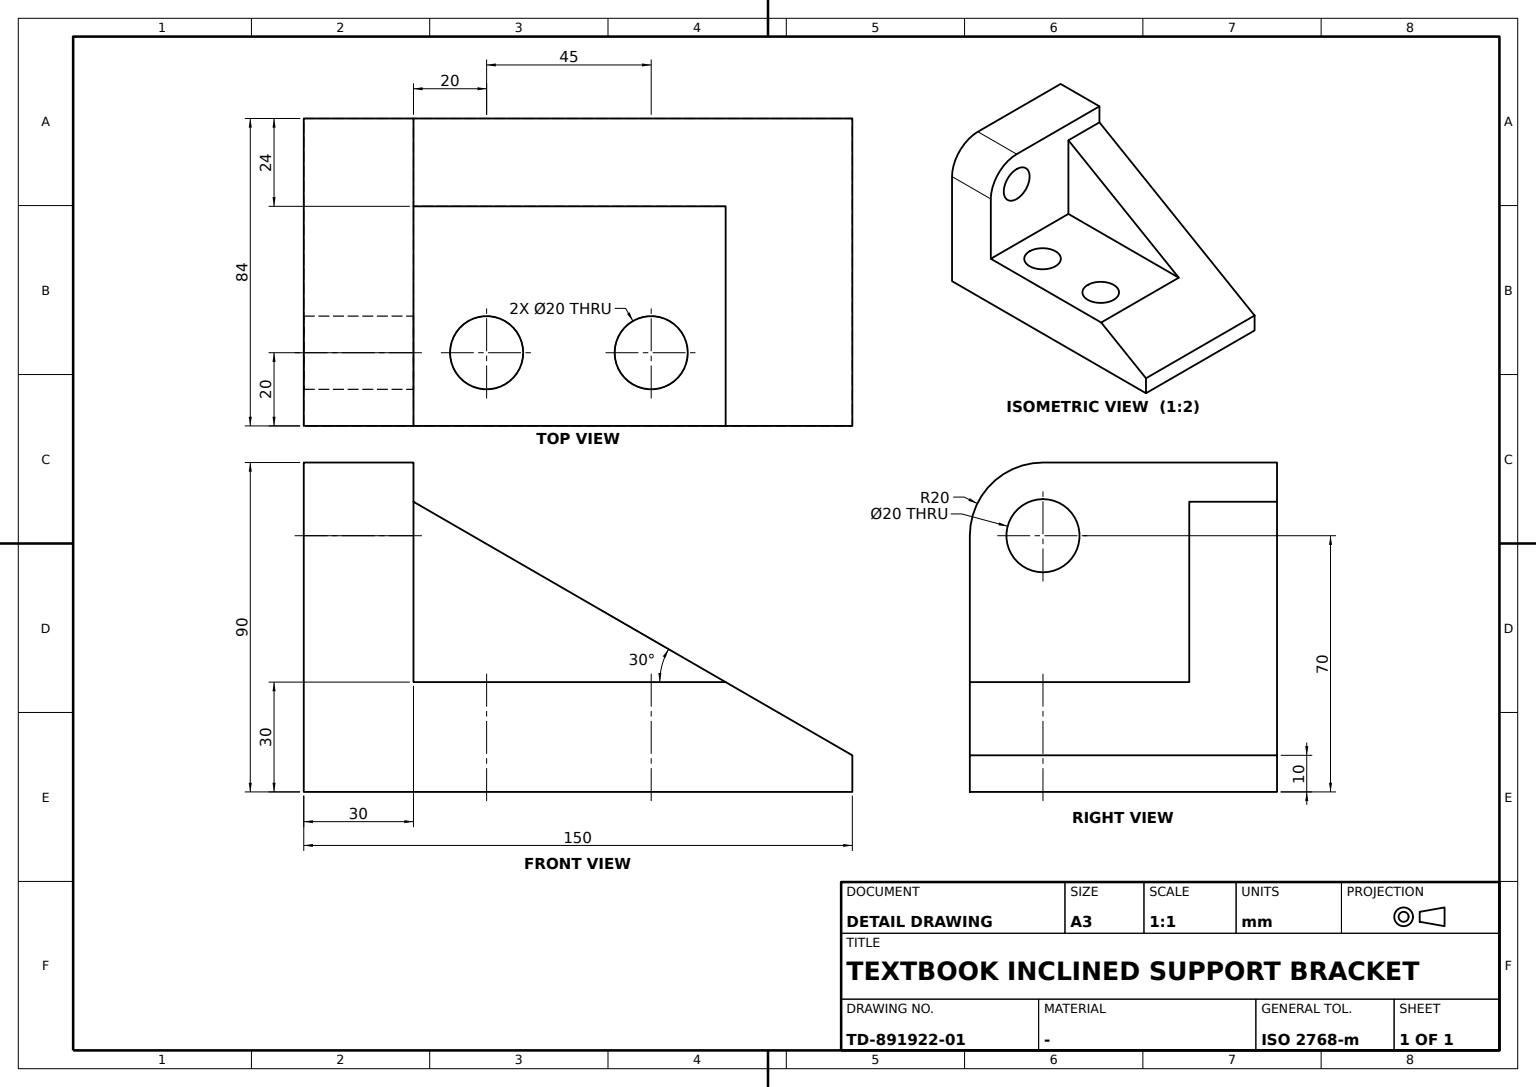
ISO-10303-21;
HEADER;
FILE_DESCRIPTION((''),'2;1');
FILE_NAME('','',(''),(''),'','','');
FILE_SCHEMA(('AUTOMOTIVE_DESIGN'));
ENDSEC;
DATA;
#1=APPLICATION_CONTEXT('');
#2=PRODUCT_CONTEXT('',#1,'mechanical');
#3=PRODUCT('','','',(#2));
#4=PRODUCT_DEFINITION_FORMATION('','',#3);
#5=PRODUCT_DEFINITION_CONTEXT('',#1,'design');
#6=PRODUCT_DEFINITION('','',#4,#5);
#7=PRODUCT_DEFINITION_SHAPE('','',#6);
#8=(LENGTH_UNIT()NAMED_UNIT(*)SI_UNIT(.MILLI.,.METRE.));
#9=(NAMED_UNIT(*)PLANE_ANGLE_UNIT()SI_UNIT($,.RADIAN.));
#10=(NAMED_UNIT(*)SI_UNIT($,.STERADIAN.)SOLID_ANGLE_UNIT());
#11=UNCERTAINTY_MEASURE_WITH_UNIT(LENGTH_MEASURE(0.005),#8,'distance_accuracy_value','');
#12=(GEOMETRIC_REPRESENTATION_CONTEXT(3)GLOBAL_UNCERTAINTY_ASSIGNED_CONTEXT((#11))GLOBAL_UNIT_ASSIGNED_CONTEXT((#8,#9,#10))REPRESENTATION_CONTEXT('',''));
#13=CARTESIAN_POINT('',(30.,-22.,60.));
#14=VERTEX_POINT('',#13);
#15=CARTESIAN_POINT('',(0.,-22.,60.));
#16=VERTEX_POINT('',#15);
#17=DIRECTION('',(1.,0.,0.));
#18=VECTOR('',#17,1000.);
#19=LINE('',#15,#18);
#20=EDGE_CURVE('',#14,#16,#19,.F.);
#21=ORIENTED_EDGE('',*,*,#20,.F.);
#22=CARTESIAN_POINT('',(30.,-22.,80.));
#23=VERTEX_POINT('',#22);
#24=CARTESIAN_POINT('',(30.,-22.,70.));
#25=DIRECTION('',(0.,1.,0.));
#26=AXIS2_PLACEMENT_3D('',#24,#17,#25);
#27=CIRCLE('',#26,10.);
#28=EDGE_CURVE('',#14,#23,#27,.T.);
#29=ORIENTED_EDGE('',*,*,#28,.T.);
#30=CARTESIAN_POINT('',(0.,-22.,80.));
#31=VERTEX_POINT('',#30);
#32=LINE('',#30,#18);
#33=EDGE_CURVE('',#31,#23,#32,.T.);
#34=ORIENTED_EDGE('',*,*,#33,.F.);
#35=CARTESIAN_POINT('',(0.,-22.,70.));
#36=AXIS2_PLACEMENT_3D('',#35,#17,#25);
#37=CIRCLE('',#36,10.);
#38=EDGE_CURVE('',#16,#31,#37,.T.);
#39=ORIENTED_EDGE('',*,*,#38,.F.);
#40=EDGE_LOOP('',(#21,#29,#34,#39));
#41=FACE_BOUND('',#40,.T.);
#42=DIRECTION('',(0.,0.,-1.));
#43=AXIS2_PLACEMENT_3D('',#35,#17,#42);
#44=CYLINDRICAL_SURFACE('',#43,10.);
#45=ADVANCED_FACE('',(#41),#44,.F.);
#46=CARTESIAN_POINT('',(85.,-22.,0.));
#47=VERTEX_POINT('',#46);
#48=CARTESIAN_POINT('',(105.,-22.,0.));
#49=VERTEX_POINT('',#48);
#50=CARTESIAN_POINT('',(95.,-22.,0.));
#51=DIRECTION('',(0.,0.,1.));
#52=AXIS2_PLACEMENT_3D('',#50,#51,#17);
#53=CIRCLE('',#52,10.);
#54=EDGE_CURVE('',#47,#49,#53,.T.);
#55=ORIENTED_EDGE('',*,*,#54,.T.);
#56=EDGE_CURVE('',#49,#47,#53,.T.);
#57=ORIENTED_EDGE('',*,*,#56,.T.);
#58=EDGE_LOOP('',(#55,#57));
#59=FACE_BOUND('',#58,.T.);
#60=CARTESIAN_POINT('',(0.,-42.,0.));
#61=VERTEX_POINT('',#60);
#62=CARTESIAN_POINT('',(0.,42.,0.));
#63=VERTEX_POINT('',#62);
#64=VECTOR('',#25,1000.);
#65=LINE('',#60,#64);
#66=EDGE_CURVE('',#61,#63,#65,.T.);
#67=ORIENTED_EDGE('',*,*,#66,.T.);
#68=CARTESIAN_POINT('',(150.,42.,0.));
#69=VERTEX_POINT('',#68);
#70=LINE('',#62,#18);
#71=EDGE_CURVE('',#63,#69,#70,.T.);
#72=ORIENTED_EDGE('',*,*,#71,.T.);
#73=CARTESIAN_POINT('',(150.,-42.,0.));
#74=VERTEX_POINT('',#73);
#75=LINE('',#73,#64);
#76=EDGE_CURVE('',#74,#69,#75,.T.);
#77=ORIENTED_EDGE('',*,*,#76,.F.);
#78=LINE('',#60,#18);
#79=EDGE_CURVE('',#61,#74,#78,.T.);
#80=ORIENTED_EDGE('',*,*,#79,.F.);
#81=EDGE_LOOP('',(#67,#72,#77,#80));
#82=FACE_BOUND('',#81,.T.);
#83=CARTESIAN_POINT('',(60.,-22.,0.));
#84=VERTEX_POINT('',#83);
#85=CARTESIAN_POINT('',(40.,-22.,0.));
#86=VERTEX_POINT('',#85);
#87=CARTESIAN_POINT('',(50.,-22.,0.));
#88=AXIS2_PLACEMENT_3D('',#87,#51,#17);
#89=CIRCLE('',#88,10.);
#90=EDGE_CURVE('',#84,#86,#89,.T.);
#91=ORIENTED_EDGE('',*,*,#90,.T.);
#92=EDGE_CURVE('',#86,#84,#89,.T.);
#93=ORIENTED_EDGE('',*,*,#92,.T.);
#94=EDGE_LOOP('',(#91,#93));
#95=FACE_BOUND('',#94,.T.);
#96=AXIS2_PLACEMENT_3D('',#60,#51,#17);
#97=PLANE('',#96);
#98=ADVANCED_FACE('',(#59,#82,#95),#97,.F.);
#99=CARTESIAN_POINT('',(30.,18.,79.282032));
#100=VERTEX_POINT('',#99);
#101=CARTESIAN_POINT('',(30.,42.,79.282032));
#102=VERTEX_POINT('',#101);
#103=LINE('',#99,#64);
#104=EDGE_CURVE('',#100,#102,#103,.T.);
#105=ORIENTED_EDGE('',*,*,#104,.F.);
#106=CARTESIAN_POINT('',(115.358984,18.,30.));
#107=VERTEX_POINT('',#106);
#108=DIRECTION('',(0.866025404,0.,-0.5));
#109=VECTOR('',#108,1000.);
#110=LINE('',#99,#109);
#111=EDGE_CURVE('',#100,#107,#110,.T.);
#112=ORIENTED_EDGE('',*,*,#111,.T.);
#113=CARTESIAN_POINT('',(115.358984,-42.,30.));
#114=VERTEX_POINT('',#113);
#115=LINE('',#113,#64);
#116=EDGE_CURVE('',#114,#107,#115,.T.);
#117=ORIENTED_EDGE('',*,*,#116,.F.);
#118=CARTESIAN_POINT('',(150.,-42.,10.));
#119=VERTEX_POINT('',#118);
#120=DIRECTION('',(-0.866025404,0.,0.5));
#121=VECTOR('',#120,1000.);
#122=LINE('',#118,#121);
#123=EDGE_CURVE('',#119,#114,#122,.T.);
#124=ORIENTED_EDGE('',*,*,#123,.F.);
#125=CARTESIAN_POINT('',(150.,42.,10.));
#126=VERTEX_POINT('',#125);
#127=LINE('',#118,#64);
#128=EDGE_CURVE('',#119,#126,#127,.T.);
#129=ORIENTED_EDGE('',*,*,#128,.T.);
#130=LINE('',#125,#121);
#131=EDGE_CURVE('',#126,#102,#130,.T.);
#132=ORIENTED_EDGE('',*,*,#131,.T.);
#133=EDGE_LOOP('',(#105,#112,#117,#124,#129,#132));
#134=FACE_BOUND('',#133,.T.);
#135=DIRECTION('',(-0.5,0.,-0.866025404));
#136=AXIS2_PLACEMENT_3D('',#118,#135,#120);
#137=PLANE('',#136);
#138=ADVANCED_FACE('',(#134),#137,.F.);
#139=ORIENTED_EDGE('',*,*,#90,.F.);
#140=CARTESIAN_POINT('',(60.,-22.,30.));
#141=VERTEX_POINT('',#140);
#142=CARTESIAN_POINT('',(60.,-22.,-54970.));
#143=VECTOR('',#51,1000.);
#144=LINE('',#142,#143);
#145=EDGE_CURVE('',#84,#141,#144,.T.);
#146=ORIENTED_EDGE('',*,*,#145,.T.);
#147=CARTESIAN_POINT('',(40.,-22.,30.));
#148=VERTEX_POINT('',#147);
#149=CARTESIAN_POINT('',(50.,-22.,30.));
#150=AXIS2_PLACEMENT_3D('',#149,#51,#17);
#151=CIRCLE('',#150,10.);
#152=EDGE_CURVE('',#141,#148,#151,.T.);
#153=ORIENTED_EDGE('',*,*,#152,.T.);
#154=CARTESIAN_POINT('',(40.,-22.,-54970.));
#155=LINE('',#154,#143);
#156=EDGE_CURVE('',#148,#86,#155,.F.);
#157=ORIENTED_EDGE('',*,*,#156,.T.);
#158=EDGE_LOOP('',(#139,#146,#153,#157));
#159=FACE_BOUND('',#158,.T.);
#160=CARTESIAN_POINT('',(50.,-22.,-54970.));
#161=AXIS2_PLACEMENT_3D('',#160,#51,#17);
#162=CYLINDRICAL_SURFACE('',#161,10.);
#163=ADVANCED_FACE('',(#159),#162,.F.);
#164=ORIENTED_EDGE('',*,*,#111,.F.);
#165=CARTESIAN_POINT('',(30.,18.,30.));
#166=VERTEX_POINT('',#165);
#167=LINE('',#165,#143);
#168=EDGE_CURVE('',#166,#100,#167,.T.);
#169=ORIENTED_EDGE('',*,*,#168,.F.);
#170=DIRECTION('',(-1.,0.,0.));
#171=VECTOR('',#170,1000.);
#172=LINE('',#106,#171);
#173=EDGE_CURVE('',#107,#166,#172,.T.);
#174=ORIENTED_EDGE('',*,*,#173,.F.);
#175=EDGE_LOOP('',(#164,#169,#174));
#176=FACE_BOUND('',#175,.T.);
#177=CARTESIAN_POINT('',(0.,18.,0.));
#178=DIRECTION('',(0.,-1.,0.));
#179=AXIS2_PLACEMENT_3D('',#177,#178,#42);
#180=PLANE('',#179);
#181=ADVANCED_FACE('',(#176),#180,.T.);
#182=CARTESIAN_POINT('',(30.,-42.,70.));
#183=VERTEX_POINT('',#182);
#184=CARTESIAN_POINT('',(0.,-42.,70.));
#185=VERTEX_POINT('',#184);
#186=LINE('',#184,#171);
#187=EDGE_CURVE('',#183,#185,#186,.T.);
#188=ORIENTED_EDGE('',*,*,#187,.F.);
#189=CARTESIAN_POINT('',(30.,-22.,90.));
#190=VERTEX_POINT('',#189);
#191=AXIS2_PLACEMENT_3D('',#24,#17,#51);
#192=CIRCLE('',#191,20.);
#193=EDGE_CURVE('',#190,#183,#192,.T.);
#194=ORIENTED_EDGE('',*,*,#193,.F.);
#195=CARTESIAN_POINT('',(0.,-22.,90.));
#196=VERTEX_POINT('',#195);
#197=LINE('',#189,#18);
#198=EDGE_CURVE('',#196,#190,#197,.T.);
#199=ORIENTED_EDGE('',*,*,#198,.F.);
#200=AXIS2_PLACEMENT_3D('',#35,#170,#42);
#201=CIRCLE('',#200,20.);
#202=EDGE_CURVE('',#185,#196,#201,.T.);
#203=ORIENTED_EDGE('',*,*,#202,.F.);
#204=EDGE_LOOP('',(#188,#194,#199,#203));
#205=FACE_BOUND('',#204,.T.);
#206=CYLINDRICAL_SURFACE('',#43,20.);
#207=ADVANCED_FACE('',(#205),#206,.T.);
#208=ORIENTED_EDGE('',*,*,#128,.F.);
#209=LINE('',#73,#143);
#210=EDGE_CURVE('',#74,#119,#209,.T.);
#211=ORIENTED_EDGE('',*,*,#210,.F.);
#212=ORIENTED_EDGE('',*,*,#76,.T.);
#213=LINE('',#68,#143);
#214=EDGE_CURVE('',#69,#126,#213,.T.);
#215=ORIENTED_EDGE('',*,*,#214,.T.);
#216=EDGE_LOOP('',(#208,#211,#212,#215));
#217=FACE_BOUND('',#216,.T.);
#218=AXIS2_PLACEMENT_3D('',#73,#170,#51);
#219=PLANE('',#218);
#220=ADVANCED_FACE('',(#217),#219,.F.);
#221=ORIENTED_EDGE('',*,*,#20,.T.);
#222=EDGE_CURVE('',#31,#16,#37,.T.);
#223=ORIENTED_EDGE('',*,*,#222,.F.);
#224=ORIENTED_EDGE('',*,*,#33,.T.);
#225=EDGE_CURVE('',#23,#14,#27,.T.);
#226=ORIENTED_EDGE('',*,*,#225,.T.);
#227=EDGE_LOOP('',(#221,#223,#224,#226));
#228=FACE_BOUND('',#227,.T.);
#229=ADVANCED_FACE('',(#228),#44,.F.);
#230=CARTESIAN_POINT('',(105.,-22.,30.));
#231=VERTEX_POINT('',#230);
#232=CARTESIAN_POINT('',(105.,-22.,-54970.));
#233=LINE('',#232,#143);
#234=EDGE_CURVE('',#49,#231,#233,.T.);
#235=ORIENTED_EDGE('',*,*,#234,.F.);
#236=ORIENTED_EDGE('',*,*,#54,.F.);
#237=CARTESIAN_POINT('',(85.,-22.,30.));
#238=VERTEX_POINT('',#237);
#239=CARTESIAN_POINT('',(85.,-22.,-54970.));
#240=LINE('',#239,#143);
#241=EDGE_CURVE('',#238,#47,#240,.F.);
#242=ORIENTED_EDGE('',*,*,#241,.F.);
#243=CARTESIAN_POINT('',(95.,-22.,30.));
#244=AXIS2_PLACEMENT_3D('',#243,#51,#17);
#245=CIRCLE('',#244,10.);
#246=EDGE_CURVE('',#238,#231,#245,.T.);
#247=ORIENTED_EDGE('',*,*,#246,.T.);
#248=EDGE_LOOP('',(#235,#236,#242,#247));
#249=FACE_BOUND('',#248,.T.);
#250=CARTESIAN_POINT('',(95.,-22.,-54970.));
#251=AXIS2_PLACEMENT_3D('',#250,#51,#17);
#252=CYLINDRICAL_SURFACE('',#251,10.);
#253=ADVANCED_FACE('',(#249),#252,.F.);
#254=CARTESIAN_POINT('',(0.,-42.,90.));
#255=VECTOR('',#42,1000.);
#256=LINE('',#254,#255);
#257=EDGE_CURVE('',#185,#61,#256,.T.);
#258=ORIENTED_EDGE('',*,*,#257,.F.);
#259=ORIENTED_EDGE('',*,*,#202,.T.);
#260=CARTESIAN_POINT('',(0.,42.,90.));
#261=VERTEX_POINT('',#260);
#262=LINE('',#254,#64);
#263=EDGE_CURVE('',#196,#261,#262,.T.);
#264=ORIENTED_EDGE('',*,*,#263,.T.);
#265=LINE('',#260,#255);
#266=EDGE_CURVE('',#261,#63,#265,.T.);
#267=ORIENTED_EDGE('',*,*,#266,.T.);
#268=ORIENTED_EDGE('',*,*,#66,.F.);
#269=EDGE_LOOP('',(#258,#259,#264,#267,#268));
#270=FACE_BOUND('',#269,.T.);
#271=ORIENTED_EDGE('',*,*,#38,.T.);
#272=ORIENTED_EDGE('',*,*,#222,.T.);
#273=EDGE_LOOP('',(#271,#272));
#274=FACE_BOUND('',#273,.T.);
#275=AXIS2_PLACEMENT_3D('',#254,#17,#42);
#276=PLANE('',#275);
#277=ADVANCED_FACE('',(#270,#274),#276,.F.);
#278=ORIENTED_EDGE('',*,*,#214,.F.);
#279=ORIENTED_EDGE('',*,*,#71,.F.);
#280=ORIENTED_EDGE('',*,*,#266,.F.);
#281=CARTESIAN_POINT('',(30.,42.,90.));
#282=VERTEX_POINT('',#281);
#283=LINE('',#281,#171);
#284=EDGE_CURVE('',#282,#261,#283,.T.);
#285=ORIENTED_EDGE('',*,*,#284,.F.);
#286=CARTESIAN_POINT('',(30.,42.,30.));
#287=LINE('',#286,#143);
#288=EDGE_CURVE('',#102,#282,#287,.T.);
#289=ORIENTED_EDGE('',*,*,#288,.F.);
#290=ORIENTED_EDGE('',*,*,#131,.F.);
#291=EDGE_LOOP('',(#278,#279,#280,#285,#289,#290));
#292=FACE_BOUND('',#291,.T.);
#293=AXIS2_PLACEMENT_3D('',#62,#178,#42);
#294=PLANE('',#293);
#295=ADVANCED_FACE('',(#292),#294,.F.);
#296=ORIENTED_EDGE('',*,*,#284,.T.);
#297=ORIENTED_EDGE('',*,*,#263,.F.);
#298=ORIENTED_EDGE('',*,*,#198,.T.);
#299=CARTESIAN_POINT('',(30.,-42.,90.));
#300=LINE('',#299,#64);
#301=EDGE_CURVE('',#190,#282,#300,.T.);
#302=ORIENTED_EDGE('',*,*,#301,.T.);
#303=EDGE_LOOP('',(#296,#297,#298,#302));
#304=FACE_BOUND('',#303,.T.);
#305=AXIS2_PLACEMENT_3D('',#299,#42,#170);
#306=PLANE('',#305);
#307=ADVANCED_FACE('',(#304),#306,.F.);
#308=ORIENTED_EDGE('',*,*,#123,.T.);
#309=CARTESIAN_POINT('',(30.,-42.,30.));
#310=VERTEX_POINT('',#309);
#311=LINE('',#113,#171);
#312=EDGE_CURVE('',#114,#310,#311,.T.);
#313=ORIENTED_EDGE('',*,*,#312,.T.);
#314=LINE('',#309,#143);
#315=EDGE_CURVE('',#310,#183,#314,.T.);
#316=ORIENTED_EDGE('',*,*,#315,.T.);
#317=ORIENTED_EDGE('',*,*,#187,.T.);
#318=ORIENTED_EDGE('',*,*,#257,.T.);
#319=ORIENTED_EDGE('',*,*,#79,.T.);
#320=ORIENTED_EDGE('',*,*,#210,.T.);
#321=EDGE_LOOP('',(#308,#313,#316,#317,#318,#319,#320));
#322=FACE_BOUND('',#321,.T.);
#323=AXIS2_PLACEMENT_3D('',#60,#178,#42);
#324=PLANE('',#323);
#325=ADVANCED_FACE('',(#322),#324,.T.);
#326=ORIENTED_EDGE('',*,*,#145,.F.);
#327=ORIENTED_EDGE('',*,*,#92,.F.);
#328=ORIENTED_EDGE('',*,*,#156,.F.);
#329=EDGE_CURVE('',#148,#141,#151,.T.);
#330=ORIENTED_EDGE('',*,*,#329,.T.);
#331=EDGE_LOOP('',(#326,#327,#328,#330));
#332=FACE_BOUND('',#331,.T.);
#333=ADVANCED_FACE('',(#332),#162,.F.);
#334=LINE('',#309,#64);
#335=EDGE_CURVE('',#310,#166,#334,.T.);
#336=ORIENTED_EDGE('',*,*,#335,.F.);
#337=ORIENTED_EDGE('',*,*,#312,.F.);
#338=ORIENTED_EDGE('',*,*,#116,.T.);
#339=ORIENTED_EDGE('',*,*,#173,.T.);
#340=EDGE_LOOP('',(#336,#337,#338,#339));
#341=FACE_BOUND('',#340,.T.);
#342=EDGE_CURVE('',#231,#238,#245,.T.);
#343=ORIENTED_EDGE('',*,*,#342,.F.);
#344=ORIENTED_EDGE('',*,*,#246,.F.);
#345=EDGE_LOOP('',(#343,#344));
#346=FACE_BOUND('',#345,.T.);
#347=ORIENTED_EDGE('',*,*,#152,.F.);
#348=ORIENTED_EDGE('',*,*,#329,.F.);
#349=EDGE_LOOP('',(#347,#348));
#350=FACE_BOUND('',#349,.T.);
#351=AXIS2_PLACEMENT_3D('',#113,#42,#170);
#352=PLANE('',#351);
#353=ADVANCED_FACE('',(#341,#346,#350),#352,.F.);
#354=ORIENTED_EDGE('',*,*,#234,.T.);
#355=ORIENTED_EDGE('',*,*,#342,.T.);
#356=ORIENTED_EDGE('',*,*,#241,.T.);
#357=ORIENTED_EDGE('',*,*,#56,.F.);
#358=EDGE_LOOP('',(#354,#355,#356,#357));
#359=FACE_BOUND('',#358,.T.);
#360=ADVANCED_FACE('',(#359),#252,.F.);
#361=ORIENTED_EDGE('',*,*,#28,.F.);
#362=ORIENTED_EDGE('',*,*,#225,.F.);
#363=EDGE_LOOP('',(#361,#362));
#364=FACE_BOUND('',#363,.T.);
#365=ORIENTED_EDGE('',*,*,#193,.T.);
#366=ORIENTED_EDGE('',*,*,#315,.F.);
#367=ORIENTED_EDGE('',*,*,#335,.T.);
#368=ORIENTED_EDGE('',*,*,#168,.T.);
#369=ORIENTED_EDGE('',*,*,#104,.T.);
#370=ORIENTED_EDGE('',*,*,#288,.T.);
#371=ORIENTED_EDGE('',*,*,#301,.F.);
#372=EDGE_LOOP('',(#365,#366,#367,#368,#369,#370,#371));
#373=FACE_BOUND('',#372,.T.);
#374=AXIS2_PLACEMENT_3D('',#309,#170,#51);
#375=PLANE('',#374);
#376=ADVANCED_FACE('',(#364,#373),#375,.F.);
#377=CLOSED_SHELL('',(#45,#98,#138,#163,#181,#207,#220,#229,#253,#277,#295,#307,#325,#333,#353,#360,#376));
#378=MANIFOLD_SOLID_BREP('',#377);
#379=ADVANCED_BREP_SHAPE_REPRESENTATION('',(#378),#12);
#380=SHAPE_DEFINITION_REPRESENTATION(#7,#379);
ENDSEC;
END-ISO-10303-21;
